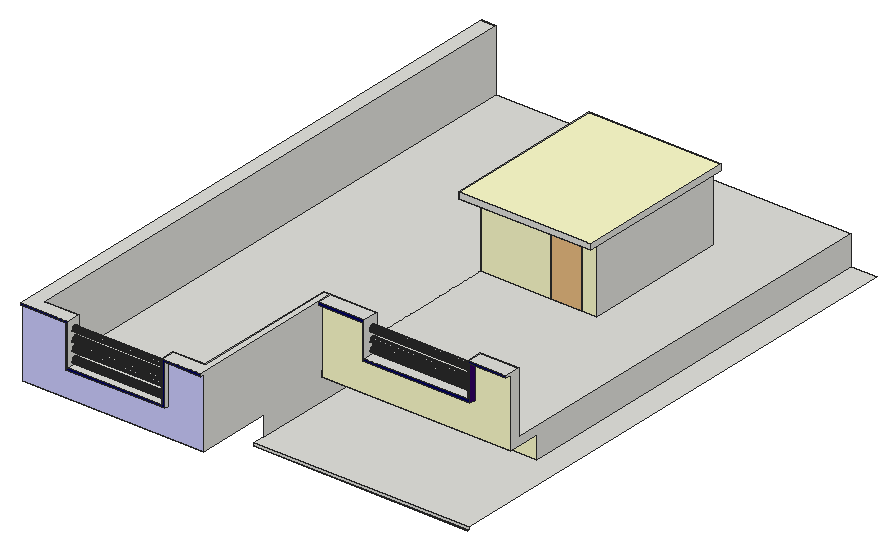
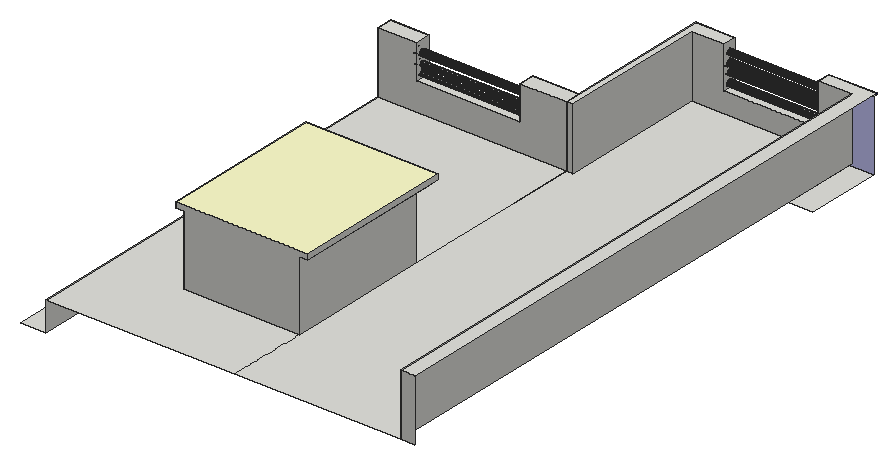
# SketchUp Ruby script. Lengths in inches.
U = 1.inch
M = Sketchup.active_model
def pt(a) = Geom::Point3d.new(a.map { |v| v * U })
def face(e, loops, mat)
  f = e.add_face(loops[0].map { |a| pt(a) })
  loops[1..].each { |l| e.add_face(l.map { |a| pt(a) }).erase! }
  f.material = f.back_material = mat if mat
  f
end
# faces: each face lists its corners as indices into pts; further lists are holes
def faces(e, pts, list, mat = nil) = list.each { |f| face(e, (f[0].is_a?(Array) ? f : [f]).map { |l| l.map { |i| pts[i] } }, mat) }
# xy, xz, yz: faces in a plane at the given z, y or x. An outline is a flat list of corners, or four numbers for a rectangle; further outlines are holes
def ring(l) = l.size == 4 ? [[l[0], l[1]], [l[2], l[1]], [l[2], l[3]], [l[0], l[3]]] : l.each_slice(2).to_a
def flat(e, list, mat, &to3) = list.each { |f| face(e, (f[0].is_a?(Array) ? f : [f]).map { |l| ring(l).map { |u, v| to3.(u, v) } }, mat) }
def xy(e, z, list, mat = nil) = flat(e, list, mat) { |x, y| [x, y, z] }
def xz(e, y, list, mat = nil) = flat(e, list, mat) { |x, z| [x, y, z] }
def yz(e, x, list, mat = nil) = flat(e, list, mat) { |y, z| [x, y, z] }
def lines(e, pts, list) = list.each { |a, b| e.add_line(pt(pts[a]), pt(pts[b])) }
# prism: a flat outline (further loops are holes) pulled along v
def prism(e, loops, v, mat = nil)
  f = face(e, loops, mat); d = Geom::Vector3d.new(v.map { |x| x * U })
  f.pushpull(f.normal.samedirection?(d) ? d.length : -d.length)
end
def box(e, o, s, mat = nil) = prism(e, [[o, [o[0] + s[0], o[1], o[2]], [o[0] + s[0], o[1] + s[1], o[2]], [o[0], o[1] + s[1], o[2]]]], [0, 0, s[2]], mat)
def at(x, y, z, deg = 0) = Geom::Transformation.translation(pt([x, y, z])) * Geom::Transformation.rotation(ORIGIN, Z_AXIS, deg.degrees)
def axes(o, x, y, z) = Geom::Transformation.new([*x, 0, *y, 0, *z, 0, *pt(o).to_a, 1])
def part(name) = M.definitions.add(name)
# library, detail: a bought-in or finely detailed component or shape, given as its bounding box
def library(name, o, s) = part(name).tap { |d| box(d.entities, o, s) }
def detail(e, o, s) = box(e.add_group.entities, o, s)
def put(e, d, t, mat = nil) = e.add_instance(d, t).tap { |i| i.material = mat if mat }
def group(e, t, mat = nil) = e.add_group.tap { |g| g.transformation = t; g.material = mat if mat }.entities
root = M.entities
M.materials.add("[Color E01]").color = [255, 255, 204]
M.materials.add("[Color I01]").color = [204, 204, 255]
M.materials.add("[Color I08]").color = [0, 0, 102]
M.materials.add("[Color J08]").color = [51, 0, 102]
M.materials.add("[Metal Corrugated Shiny]").color = [193, 193, 193]
c1 = library("Untitled (1)",[0,0,0],[36,4.39,84])
xy(root,523.46,[[2058.38,1123.42,2631.21,1124.92]])
xy(root,530.44,[[2058.38,1124.92,2631.21,1124.92,2631.21,2487.49,2562.14,2487.49,2562.14,1439.1875,2058.38,1439.1875]])
xy(root,584.23,[[1576.31,956.92,2058.38,1158.61]])
xy(root,590.17,[[2058.38,1351.75,2562.14,1439.1875]])
xy(root,609.375,[[1613.64,984,2040.63,984,2040.63,1379.78,2058.38,1379.78,2058.38,2487.49,1613.64,2487.49],[2058.38,1379.78,2562.14,1379.78,2562.14,2487.49,2058.38,2487.49,2058.38,2271.7,2367.06,2271.7,2367.06,1882.82,2329.3,1882.82,2329.3,1931.82,2244.36,1931.82,2244.36,1882.82,2058.38,1882.82]])
xy(root,657.8,[[1697.13,947.29,1961.38,956.92]])
xy(root,663.8125,[[1703.3,947.29,1955.43,984]])
xy(root,676.26,[[2178.19,1337.75,2465.88,1351.75]],"[Color J08]")
xy(root,682.75,[[2182.45,1337.75,2459.18,1379.78]])
xy(root,766.82,[[2058.38,1337.75,2178.19,1351.75]],"[Color J08]")
xy(root,767.87,[[1961.38,947.29,2049.45,956.92],[2049.45,947.29,2058.38,956.92]])
xy(root,769.01,[[2465.88,1337.75,2562.14,1351.75]])
xy(root,769.62,[[1576.31,947.29,1697.13,956.92]])
xy(root,774.9375,[[1576.31,947.29,1703.3,947.29,1703.3,984,1613.64,984,1613.64,2487.49,1576.31,2487.49],[1955.43,947.29,2058.38,947.29,2058.38,1379.78,2040.63,1379.78,2040.63,984,1955.43,984],[2058.38,1337.75,2182.45,1379.78],[2459.18,1337.75,2562.14,1379.78]])
xy(root,777.125,[[2244.36,1882.82,2329.3,1931.82]])
xy(root,795.49,[[2035.81,1837.14,2367.06,1882.82],[2367.06,1837.14,2388.25,2271.7],[2035.81,1882.82,2058.38,2271.7]])
xy(root,811.0625,[[2035.81,1837.14,2388.25,2271.7]],"[Color E01]")
xz(root,947.29,[[1697.13,657.8,1961.38,657.8,1961.38,767.87,2058.38,767.87,2058.38,774.9375,1955.43,774.9375,1955.43,663.8125,1703.3,663.8125,1703.3,774.9375,1576.31,774.9375,1576.31,769.62,1697.13,769.62]],"[Color I08]")
xz(root,956.92,[[1576.31,584.23,2058.38,584.23,2058.38,767.87,1961.38,767.87,1961.38,657.8,1697.13,657.8,1697.13,769.62,1576.31,769.62]],"[Color I01]")
xz(root,984,[[1613.64,609.375,1613.64,774.9375,1703.3,774.9375,1703.3,663.8125,1955.43,663.8125,1955.43,774.9375,2040.63,774.9375,2040.63,609.375]])
xz(root,1124.92,[[2058.38,523.46,2631.21,530.44]])
xz(root,1337.75,[[2178.19,676.26,2465.88,676.26,2465.88,769.01,2562.14,769.01,2562.14,774.9375,2459.18,774.9375,2459.18,682.75,2182.45,682.75,2182.45,774.9375,2058.38,774.9375,2058.38,766.82,2178.19,766.82]],"[Color I08]")
xz(root,1351.75,[[2058.38,590.17,2562.14,590.17,2562.14,769.01,2465.88,769.01,2465.88,676.26,2178.19,676.26,2178.19,766.82,2058.38,766.82]],"[Color E01]")
xz(root,1379.78,[[2040.63,609.375,2058.38,774.9375],[2058.38,609.375,2058.38,774.9375,2182.45,774.9375,2182.45,682.75,2459.18,682.75,2459.18,774.9375,2562.14,774.9375,2562.14,609.375]])
xz(root,1439.1875,[[2058.38,530.44,2562.14,590.17]],"[Color E01]")
xz(root,1837.14,[[2035.81,795.49,2388.25,811.0625]])
xz(root,1882.82,[[2058.38,609.375,2244.36,609.375,2244.36,777.125,2329.3,777.125,2329.3,609.375,2367.06,609.375,2367.06,795.49,2058.38,795.49]],"[Color E01]")
xz(root,1931.82,[[2244.36,609.375,2329.3,777.125]])
xz(root,2271.7,[[2058.38,609.375,2058.38,795.49,2035.81,795.49,2035.81,811.0625,2388.25,811.0625,2388.25,795.49,2367.06,795.49,2367.06,609.375]])
xz(root,2487.49,[[1576.31,609.375,1613.64,774.9375]])
yz(root,1613.64,[[984,609.375,2487.49,774.9375]])
yz(root,1697.13,[[947.29,657.8,956.92,769.62]])
yz(root,1703.3,[[[947.29,663.8125,984,774.9375],[966.94,667.97,964.95,668.23,963.1,669,961.51,670.22,960.28,671.8125,959.52,673.67,959.26,675.66,959.52,677.65,960.28,679.5,961.51,681.09,963.1,682.32,964.95,683.08,966.94,683.35,968.93,683.08,970.79,682.32,972.38,681.09,973.6,679.5,974.37,677.65,974.63,675.66,974.37,673.67,973.6,671.8125,972.38,670.22,970.79,669,968.93,668.23],[966.94,717.85,964.99,718.11,963.16,718.86,961.6,720.07,960.39,721.63,959.64,723.46,959.38,725.41,959.64,727.37,960.39,729.19,961.6,730.76,963.16,731.96,964.99,732.72,966.94,732.98,968.9,732.72,970.72,731.96,972.29,730.76,973.49,729.19,974.25,727.37,974.51,725.41,974.25,723.46,973.49,721.63,972.29,720.07,970.72,718.86,968.9,718.11],[966.94,695.32,965.1,695.56,963.38,696.27,961.9,697.4,960.77,698.88,960.06,700.6,959.82,702.44,960.06,704.29,960.77,706,961.9,707.48,963.38,708.61,965.1,709.32,966.94,709.57,968.79,709.32,970.51,708.61,971.98,707.48,973.11,706,973.82,704.29,974.07,702.44,973.82,700.6,973.11,698.88,971.98,697.4,970.51,696.27,968.79,695.56],[966.94,743.37,965.16,743.6,963.51,744.29,962.08,745.38,960.99,746.81,960.3,748.46,960.07,750.24,960.3,752.02,960.99,753.68,962.08,755.11,963.51,756.2,965.16,756.88,966.94,757.12,968.72,756.88,970.38,756.2,971.8,755.11,972.9,753.68,973.58,752.02,973.82,750.24,973.58,748.46,972.9,746.81,971.8,745.38,970.38,744.29,968.72,743.6]]])
yz(root,1954.62,[[966.94,667.97,968.93,668.23,970.79,669,972.38,670.22,973.6,671.8125,974.37,673.67,974.63,675.66,974.37,677.65,973.6,679.5,972.38,681.09,970.79,682.32,968.93,683.08,966.94,683.35,964.95,683.08,963.1,682.32,961.51,681.09,960.28,679.5,959.52,677.65,959.26,675.66,959.52,673.67,960.28,671.8125,961.51,670.22,963.1,669,964.95,668.23]])
yz(root,1955.43,[[[947.29,663.8125,984,774.9375],[966.94,717.85,968.9,718.11,970.72,718.86,972.29,720.07,973.49,721.63,974.25,723.46,974.51,725.41,974.25,727.37,973.49,729.19,972.29,730.76,970.72,731.96,968.9,732.72,966.94,732.98,964.99,732.72,963.16,731.96,961.6,730.76,960.39,729.19,959.64,727.37,959.38,725.41,959.64,723.46,960.39,721.63,961.6,720.07,963.16,718.86,964.99,718.11],[966.94,743.37,968.72,743.6,970.38,744.29,971.8,745.38,972.9,746.81,973.58,748.46,973.82,750.24,973.58,752.02,972.9,753.68,971.8,755.11,970.38,756.2,968.72,756.88,966.94,757.12,965.16,756.88,963.51,756.2,962.08,755.11,960.99,753.68,960.3,752.02,960.07,750.24,960.3,748.46,960.99,746.81,962.08,745.38,963.51,744.29,965.16,743.6]]])
yz(root,1961.38,[[947.29,657.8,956.92,767.87]])
yz(root,1968.7,[[966.94,695.32,968.79,695.56,970.51,696.27,971.98,697.4,973.11,698.88,973.82,700.6,974.07,702.44,973.82,704.29,973.11,706,971.98,707.48,970.51,708.61,968.79,709.32,966.94,709.57,965.1,709.32,963.38,708.61,961.9,707.48,960.77,706,960.06,704.29,959.82,702.44,960.06,700.6,960.77,698.88,961.9,697.4,963.38,696.27,965.1,695.56]])
yz(root,2035.81,[[1837.14,795.49,2271.7,811.0625]])
yz(root,2040.63,[[984,609.375,1379.78,774.9375]])
yz(root,2058.38,[[1158.61,530.44,1439.1875,530.44,1439.1875,590.17,1351.75,590.17,1351.75,766.82,1337.75,766.82,1337.75,774.9375,947.29,774.9375,947.29,767.87,956.92,767.87,956.92,584.23,1158.61,584.23],[1439.1875,530.44,1553.21,530.44,1553.21,609.375,1351.75,609.375,1351.75,590.17,1439.1875,590.17],[1351.75,609.375,1379.78,609.375,1379.78,774.9375,1337.75,774.9375,1337.75,766.82,1351.75,766.82],[1882.82,609.375,2271.7,795.49]])
yz(root,2178.19,[[1337.75,676.26,1351.75,766.82]],"[Color J08]")
yz(root,2182.45,[[[1337.75,682.75,1379.78,774.9375],[1362.9375,737.56,1360.71,737.85,1358.625,738.71,1356.84,740.08,1355.47,741.87,1354.61,743.95,1354.3125,746.18,1354.61,748.42,1355.47,750.5,1356.84,752.28,1358.625,753.65,1360.71,754.51,1362.9375,754.81,1365.17,754.51,1367.25,753.65,1369.04,752.28,1370.41,750.5,1371.27,748.42,1371.5625,746.18,1371.27,743.95,1370.41,741.87,1369.04,740.08,1367.25,738.71,1365.17,737.85],[1362.9375,689.17,1361.08,689.42,1359.34,690.14,1357.86,691.28,1356.71,692.77,1356,694.5,1355.75,696.36,1356,698.22,1356.71,699.95,1357.86,701.44,1359.34,702.59,1361.08,703.3,1362.9375,703.55,1364.8,703.3,1366.53,702.59,1368.02,701.44,1369.16,699.95,1369.88,698.22,1370.125,696.36,1369.88,694.5,1369.16,692.77,1368.02,691.28,1366.53,690.14,1364.8,689.42],[1362.9375,711.99,1361.09,712.23,1359.375,712.94,1357.9,714.07,1356.77,715.55,1356.06,717.27,1355.8125,719.11,1356.06,720.95,1356.77,722.67,1357.9,724.15,1359.375,725.28,1361.09,725.99,1362.9375,726.24,1364.78,725.99,1366.5,725.28,1367.98,724.15,1369.11,722.67,1369.82,720.95,1370.0625,719.11,1369.82,717.27,1369.11,715.55,1367.98,714.07,1366.5,712.94,1364.78,712.23]]])
yz(root,2244.36,[[1882.82,609.375,1931.82,777.125]])
yz(root,2329.3,[[1882.82,609.375,1931.82,777.125]])
yz(root,2367.06,[[1882.82,609.375,2271.7,795.49]])
yz(root,2388.25,[[1837.14,795.49,2271.7,811.0625]])
yz(root,2459.18,[[1337.75,682.75,1379.78,774.9375]])
yz(root,2462.64,[[1362.9375,689.17,1364.8,689.42,1366.53,690.14,1368.02,691.28,1369.16,692.77,1369.88,694.5,1370.125,696.36,1369.88,698.22,1369.16,699.95,1368.02,701.44,1366.53,702.59,1364.8,703.3,1362.9375,703.55,1361.08,703.3,1359.34,702.59,1357.86,701.44,1356.71,699.95,1356,698.22,1355.75,696.36,1356,694.5,1356.71,692.77,1357.86,691.28,1359.34,690.14,1361.08,689.42]])
yz(root,2465.88,[[1337.75,676.26,1351.75,769.01]],"[Color J08]")
yz(root,2475.75,[[1362.9375,711.99,1364.78,712.23,1366.5,712.94,1367.98,714.07,1369.11,715.55,1369.82,717.27,1370.0625,719.11,1369.82,720.95,1369.11,722.67,1367.98,724.15,1366.5,725.28,1364.78,725.99,1362.9375,726.24,1361.09,725.99,1359.375,725.28,1357.9,724.15,1356.77,722.67,1356.06,720.95,1355.8125,719.11,1356.06,717.27,1356.77,715.55,1357.9,714.07,1359.375,712.94,1361.09,712.23],[1362.9375,737.56,1365.17,737.85,1367.25,738.71,1369.04,740.08,1370.41,741.87,1371.27,743.95,1371.5625,746.18,1371.27,748.42,1370.41,750.5,1369.04,752.28,1367.25,753.65,1365.17,754.51,1362.9375,754.81,1360.71,754.51,1358.625,753.65,1356.84,752.28,1355.47,750.5,1354.61,748.42,1354.3125,746.18,1354.61,743.95,1355.47,741.87,1356.84,740.08,1358.625,738.71,1360.71,737.85]])
yz(root,2562.14,[[1439.1875,530.44,2487.49,530.44,2487.49,609.375,1379.78,609.375,1379.78,774.9375,1337.75,774.9375,1337.75,769.01,1351.75,769.01,1351.75,590.17,1439.1875,590.17]])
p = [[1703.3,964.95,668.23],[1703.3,966.94,667.97],[1954.62,966.94,667.97],[1954.62,964.95,668.23],[1703.3,968.93,668.23],[1954.62,968.93,668.23],
  [1703.3,963.1,669],[1954.62,963.1,669],[1703.3,970.79,669],[1954.62,970.79,669],[1703.3,961.51,670.22],[1954.62,961.51,670.22],
  [1703.3,972.38,670.22],[1954.62,972.38,670.22],[1703.3,960.28,671.8125],[1954.62,960.28,671.8125],[1703.3,973.6,671.8125],[1954.62,973.6,671.8125],
  [1703.3,959.52,673.67],[1954.62,959.52,673.67],[1703.3,974.37,673.67],[1954.62,974.37,673.67],[1703.3,959.26,675.66],[1954.62,959.26,675.66],
  [1703.3,974.63,675.66],[1954.62,974.63,675.66],[1703.3,959.52,677.65],[1954.62,959.52,677.65],[1703.3,974.37,677.65],[1954.62,974.37,677.65],
  [1703.3,960.28,679.5],[1954.62,960.28,679.5],[1703.3,973.6,679.5],[1954.62,973.6,679.5],[1703.3,961.51,681.09],[1954.62,961.51,681.09],
  [1703.3,972.38,681.09],[1954.62,972.38,681.09],[1703.3,963.1,682.32],[1954.62,963.1,682.32],[1703.3,970.79,682.32],[1954.62,970.79,682.32],
  [1703.3,964.95,683.08],[1954.62,964.95,683.08],[1703.3,968.93,683.08],[1954.62,968.93,683.08],[1703.3,966.94,683.35],[1954.62,966.94,683.35],
  [2182.45,1361.08,689.42],[2182.45,1362.9375,689.17],[2462.64,1362.9375,689.17],[2462.64,1361.08,689.42],[2182.45,1364.8,689.42],[2462.64,1364.8,689.42],
  [2182.45,1359.34,690.14],[2462.64,1359.34,690.14],[2182.45,1366.53,690.14],[2462.64,1366.53,690.14],[2182.45,1357.86,691.28],[2462.64,1357.86,691.28],
  [2182.45,1368.02,691.28],[2462.64,1368.02,691.28],[2182.45,1356.71,692.77],[2462.64,1356.71,692.77],[2182.45,1369.16,692.77],[2462.64,1369.16,692.77],
  [2182.45,1356,694.5],[2462.64,1356,694.5],[2182.45,1369.88,694.5],[2462.64,1369.88,694.5],[2182.45,1355.75,696.36],[2462.64,1355.75,696.36],
  [2182.45,1370.125,696.36],[2462.64,1370.125,696.36],[1703.3,965.1,695.56],[1703.3,966.94,695.32],[1968.7,966.94,695.32],[1968.7,965.1,695.56],
  [1703.3,968.79,695.56],[1968.7,968.79,695.56],[1703.3,963.38,696.27],[1968.7,963.38,696.27],[1703.3,970.51,696.27],[1968.7,970.51,696.27],
  [1703.3,961.9,697.4],[1968.7,961.9,697.4],[1703.3,971.98,697.4],[1968.7,971.98,697.4],[2182.45,1356,698.22],[2462.64,1356,698.22],
  [2182.45,1369.88,698.22],[2462.64,1369.88,698.22],[1703.3,960.77,698.88],[1968.7,960.77,698.88],[1703.3,973.11,698.88],[1968.7,973.11,698.88],
  [2182.45,1356.71,699.95],[2462.64,1356.71,699.95],[2182.45,1369.16,699.95],[2462.64,1369.16,699.95],[1703.3,960.06,700.6],[1968.7,960.06,700.6],
  [1703.3,973.82,700.6],[1968.7,973.82,700.6],[2182.45,1357.86,701.44],[2462.64,1357.86,701.44],[2182.45,1368.02,701.44],[2462.64,1368.02,701.44],
  [1703.3,959.82,702.44],[1968.7,959.82,702.44],[1703.3,974.07,702.44],[1968.7,974.07,702.44],[2182.45,1359.34,702.59],[2462.64,1359.34,702.59],
  [2182.45,1366.53,702.59],[2462.64,1366.53,702.59],[1703.3,960.06,704.29],[1968.7,960.06,704.29],[1703.3,973.82,704.29],[1968.7,973.82,704.29],
  [2182.45,1361.08,703.3],[2462.64,1361.08,703.3],[2182.45,1364.8,703.3],[2462.64,1364.8,703.3],[2182.45,1362.9375,703.55],[2462.64,1362.9375,703.55],
  [1703.3,960.77,706],[1968.7,960.77,706],[1703.3,973.11,706],[1968.7,973.11,706],[1703.3,961.9,707.48],[1968.7,961.9,707.48],
  [1703.3,971.98,707.48],[1968.7,971.98,707.48],[1703.3,963.38,708.61],[1968.7,963.38,708.61],[1703.3,970.51,708.61],[1968.7,970.51,708.61],
  [1703.3,965.1,709.32],[1968.7,965.1,709.32],[1703.3,968.79,709.32],[1968.7,968.79,709.32],[1703.3,966.94,709.57],[1968.7,966.94,709.57],
  [2182.45,1361.09,712.23],[2182.45,1362.9375,711.99],[2475.75,1362.9375,711.99],[2475.75,1361.09,712.23],[2182.45,1364.78,712.23],[2475.75,1364.78,712.23],
  [2182.45,1359.375,712.94],[2475.75,1359.375,712.94],[2182.45,1366.5,712.94],[2475.75,1366.5,712.94],[2182.45,1357.9,714.07],[2475.75,1357.9,714.07],
  [2182.45,1367.98,714.07],[2475.75,1367.98,714.07],[2182.45,1356.77,715.55],[2475.75,1356.77,715.55],[2182.45,1369.11,715.55],[2475.75,1369.11,715.55],
  [2182.45,1356.06,717.27],[2475.75,1356.06,717.27],[2182.45,1369.82,717.27],[2475.75,1369.82,717.27],[2182.45,1355.8125,719.11],[2475.75,1355.8125,719.11],
  [2182.45,1370.0625,719.11],[2475.75,1370.0625,719.11],[1703.3,964.99,718.11],[1703.3,966.94,717.85],[1955.43,966.94,717.85],[1955.43,964.99,718.11],
  [1703.3,968.9,718.11],[1955.43,968.9,718.11],[1703.3,963.16,718.86],[1955.43,963.16,718.86],[1703.3,970.72,718.86],[1955.43,970.72,718.86],
  [1703.3,961.6,720.07],[1955.43,961.6,720.07],[1703.3,972.29,720.07],[1955.43,972.29,720.07],[2182.45,1356.06,720.95],[2475.75,1356.06,720.95],
  [2182.45,1369.82,720.95],[2475.75,1369.82,720.95],[1703.3,960.39,721.63],[1955.43,960.39,721.63],[1703.3,973.49,721.63],[1955.43,973.49,721.63],
  [2182.45,1356.77,722.67],[2475.75,1356.77,722.67],[2182.45,1369.11,722.67],[2475.75,1369.11,722.67],[1703.3,959.64,723.46],[1955.43,959.64,723.46],
  [1703.3,974.25,723.46],[1955.43,974.25,723.46],[2182.45,1357.9,724.15],[2475.75,1357.9,724.15],[2182.45,1367.98,724.15],[2475.75,1367.98,724.15],
  [1703.3,959.38,725.41],[1955.43,959.38,725.41],[1703.3,974.51,725.41],[1955.43,974.51,725.41],[2182.45,1359.375,725.28],[2475.75,1359.375,725.28],
  [2182.45,1366.5,725.28],[2475.75,1366.5,725.28],[2182.45,1361.09,725.99],[2475.75,1361.09,725.99],[2182.45,1364.78,725.99],[2475.75,1364.78,725.99],
  [1703.3,959.64,727.37],[1955.43,959.64,727.37],[1703.3,974.25,727.37],[1955.43,974.25,727.37],[2182.45,1362.9375,726.24],[2475.75,1362.9375,726.24],
  [1703.3,960.39,729.19],[1955.43,960.39,729.19],[1703.3,973.49,729.19],[1955.43,973.49,729.19],[1703.3,961.6,730.76],[1955.43,961.6,730.76],
  [1703.3,972.29,730.76],[1955.43,972.29,730.76],[1703.3,963.16,731.96],[1955.43,963.16,731.96],[1703.3,970.72,731.96],[1955.43,970.72,731.96],
  [1703.3,964.99,732.72],[1955.43,964.99,732.72],[1703.3,968.9,732.72],[1955.43,968.9,732.72],[1703.3,966.94,732.98],[1955.43,966.94,732.98],
  [2182.45,1360.71,737.85],[2182.45,1362.9375,737.56],[2475.75,1362.9375,737.56],[2475.75,1360.71,737.85],[2182.45,1365.17,737.85],[2475.75,1365.17,737.85],
  [2182.45,1358.625,738.71],[2475.75,1358.625,738.71],[2182.45,1367.25,738.71],[2475.75,1367.25,738.71],[2182.45,1356.84,740.08],[2475.75,1356.84,740.08],
  [2182.45,1369.04,740.08],[2475.75,1369.04,740.08],[2182.45,1355.47,741.87],[2475.75,1355.47,741.87],[2182.45,1370.41,741.87],[2475.75,1370.41,741.87],
  [2182.45,1354.61,743.95],[2475.75,1354.61,743.95],[2182.45,1371.27,743.95],[2475.75,1371.27,743.95],[1703.3,965.16,743.6],[1703.3,966.94,743.37],
  [1955.43,966.94,743.37],[1955.43,965.16,743.6],[1703.3,968.72,743.6],[1955.43,968.72,743.6],[1703.3,963.51,744.29],[1955.43,963.51,744.29],
  [1703.3,970.38,744.29],[1955.43,970.38,744.29],[2182.45,1354.3125,746.18],[2475.75,1354.3125,746.18],[2182.45,1371.5625,746.18],[2475.75,1371.5625,746.18],
  [1703.3,962.08,745.38],[1955.43,962.08,745.38],[1703.3,971.8,745.38],[1955.43,971.8,745.38],[1703.3,960.99,746.81],[1955.43,960.99,746.81],
  [1703.3,972.9,746.81],[1955.43,972.9,746.81],[2182.45,1354.61,748.42],[2475.75,1354.61,748.42],[2182.45,1371.27,748.42],[2475.75,1371.27,748.42],
  [1703.3,960.3,748.46],[1955.43,960.3,748.46],[1703.3,973.58,748.46],[1955.43,973.58,748.46],[2182.45,1355.47,750.5],[2475.75,1355.47,750.5],
  [2182.45,1370.41,750.5],[2475.75,1370.41,750.5],[1703.3,960.07,750.24],[1955.43,960.07,750.24],[1703.3,973.82,750.24],[1955.43,973.82,750.24],
  [1703.3,960.3,752.02],[1955.43,960.3,752.02],[1703.3,973.58,752.02],[1955.43,973.58,752.02],[2182.45,1356.84,752.28],[2475.75,1356.84,752.28],
  [2182.45,1369.04,752.28],[2475.75,1369.04,752.28],[1703.3,960.99,753.68],[1955.43,960.99,753.68],[1703.3,972.9,753.68],[1955.43,972.9,753.68],
  [2182.45,1358.625,753.65],[2475.75,1358.625,753.65],[2182.45,1367.25,753.65],[2475.75,1367.25,753.65],[1703.3,962.08,755.11],[1955.43,962.08,755.11],
  [1703.3,971.8,755.11],[1955.43,971.8,755.11],[2182.45,1360.71,754.51],[2475.75,1360.71,754.51],[2182.45,1365.17,754.51],[2475.75,1365.17,754.51],
  [2182.45,1362.9375,754.81],[2475.75,1362.9375,754.81],[1703.3,963.51,756.2],[1955.43,963.51,756.2],[1703.3,970.38,756.2],[1955.43,970.38,756.2],
  [1703.3,965.16,756.88],[1955.43,965.16,756.88],[1703.3,968.72,756.88],[1955.43,968.72,756.88],[1703.3,966.94,757.12],[1955.43,966.94,757.12]]
faces(root,p,[[0,1,2,3],[1,4,5,2],[6,0,3,7],[4,8,9,5],[10,6,7,11],[8,12,13,9],[14,10,11,15],[12,16,17,13],
  [18,14,15,19],[16,20,21,17],[22,18,19,23],[20,24,25,21],[26,22,23,27],[24,28,29,25],[30,26,27,31],[28,32,33,29],
  [34,30,31,35],[32,36,37,33],[38,34,35,39],[36,40,41,37],[42,38,39,43],[40,44,45,41],[46,42,43,47],[44,46,47,45],
  [48,49,50,51],[49,52,53,50],[54,48,51,55],[52,56,57,53],[58,54,55,59],[56,60,61,57],[62,58,59,63],[60,64,65,61],
  [66,62,63,67],[64,68,69,65],[70,66,67,71],[68,72,73,69],[74,75,76,77],[75,78,79,76],[80,74,77,81],[78,82,83,79],
  [84,80,81,85],[82,86,87,83],[88,70,71,89],[72,90,91,73],[92,84,85,93],[86,94,95,87],[96,88,89,97],[90,98,99,91],
  [100,92,93,101],[94,102,103,95],[104,96,97,105],[98,106,107,99],[108,100,101,109],[102,110,111,103],[112,104,105,113],[106,114,115,107],
  [116,108,109,117],[110,118,119,111],[120,112,113,121],[114,122,123,115],[124,120,121,125],[122,124,125,123],[126,116,117,127],[118,128,129,119],
  [130,126,127,131],[128,132,133,129],[134,130,131,135],[132,136,137,133],[138,134,135,139],[136,140,141,137],[142,138,139,143],[140,142,143,141],
  [144,145,146,147],[145,148,149,146],[150,144,147,151],[148,152,153,149],[154,150,151,155],[152,156,157,153],[158,154,155,159],[156,160,161,157],
  [162,158,159,163],[160,164,165,161],[166,162,163,167],[164,168,169,165],[170,171,172,173],[171,174,175,172],[176,170,173,177],[174,178,179,175],
  [180,176,177,181],[178,182,183,179],[184,166,167,185],[168,186,187,169],[188,180,181,189],[182,190,191,183],[192,184,185,193],[186,194,195,187],
  [196,188,189,197],[190,198,199,191],[200,192,193,201],[194,202,203,195],[204,196,197,205],[198,206,207,199],[208,200,201,209],[202,210,211,203],
  [212,208,209,213],[210,214,215,211],[216,204,205,217],[206,218,219,207],[220,212,213,221],[214,220,221,215],[222,216,217,223],[218,224,225,219],
  [226,222,223,227],[224,228,229,225],[230,226,227,231],[228,232,233,229],[234,230,231,235],[232,236,237,233],[238,234,235,239],[236,238,239,237],
  [240,241,242,243],[241,244,245,242],[246,240,243,247],[244,248,249,245],[250,246,247,251],[248,252,253,249],[254,250,251,255],[252,256,257,253],
  [258,254,255,259],[256,260,261,257],[262,263,264,265],[263,266,267,264],[268,262,265,269],[266,270,271,267],[272,258,259,273],[260,274,275,261],
  [276,268,269,277],[270,278,279,271],[280,276,277,281],[278,282,283,279],[284,272,273,285],[274,286,287,275],[288,280,281,289],[282,290,291,283],
  [292,284,285,293],[286,294,295,287],[296,288,289,297],[290,298,299,291],[300,296,297,301],[298,302,303,299],[304,292,293,305],[294,306,307,295],
  [308,300,301,309],[302,310,311,303],[312,304,305,313],[306,314,315,307],[316,308,309,317],[310,318,319,311],[320,312,313,321],[314,322,323,315],
  [324,320,321,325],[322,324,325,323],[326,316,317,327],[318,328,329,319],[330,326,327,331],[328,332,333,329],[334,330,331,335],[332,334,335,333]],"[Metal Corrugated Shiny]")
put(root,c1,axes([2244.36,1882.82,609.375],[2.35937,0,0],[0,4.7128,0],[0,0,1.99702]))
